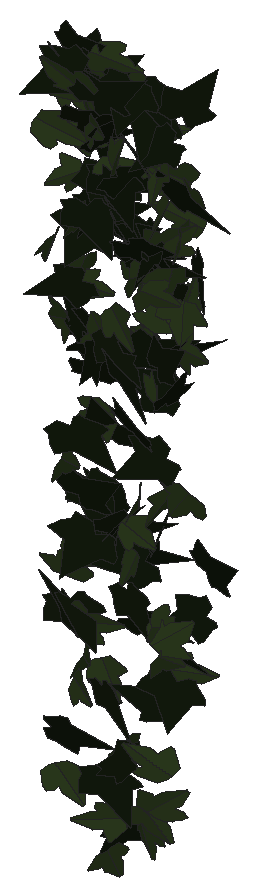
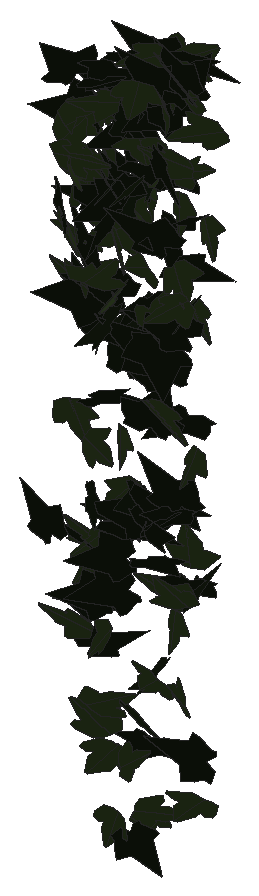
# SketchUp Ruby script. Lengths in inches.
U = 1.inch
M = Sketchup.active_model
def pt(a) = Geom::Point3d.new(a.map { |v| v * U })
def face(e, loops, mat)
  f = e.add_face(loops[0].map { |a| pt(a) })
  loops[1..].each { |l| e.add_face(l.map { |a| pt(a) }).erase! }
  f.material = f.back_material = mat if mat
  f
end
# faces: each face lists its corners as indices into pts; further lists are holes
def faces(e, pts, list, mat = nil) = list.each { |f| face(e, (f[0].is_a?(Array) ? f : [f]).map { |l| l.map { |i| pts[i] } }, mat) }
# xy, xz, yz: faces in a plane at the given z, y or x. An outline is a flat list of corners, or four numbers for a rectangle; further outlines are holes
def ring(l) = l.size == 4 ? [[l[0], l[1]], [l[2], l[1]], [l[2], l[3]], [l[0], l[3]]] : l.each_slice(2).to_a
def flat(e, list, mat, &to3) = list.each { |f| face(e, (f[0].is_a?(Array) ? f : [f]).map { |l| ring(l).map { |u, v| to3.(u, v) } }, mat) }
def xy(e, z, list, mat = nil) = flat(e, list, mat) { |x, y| [x, y, z] }
def xz(e, y, list, mat = nil) = flat(e, list, mat) { |x, z| [x, y, z] }
def yz(e, x, list, mat = nil) = flat(e, list, mat) { |y, z| [x, y, z] }
def lines(e, pts, list) = list.each { |a, b| e.add_line(pt(pts[a]), pt(pts[b])) }
# prism: a flat outline (further loops are holes) pulled along v
def prism(e, loops, v, mat = nil)
  f = face(e, loops, mat); d = Geom::Vector3d.new(v.map { |x| x * U })
  f.pushpull(f.normal.samedirection?(d) ? d.length : -d.length)
end
def box(e, o, s, mat = nil) = prism(e, [[o, [o[0] + s[0], o[1], o[2]], [o[0] + s[0], o[1] + s[1], o[2]], [o[0], o[1] + s[1], o[2]]]], [0, 0, s[2]], mat)
def at(x, y, z, deg = 0) = Geom::Transformation.translation(pt([x, y, z])) * Geom::Transformation.rotation(ORIGIN, Z_AXIS, deg.degrees)
def axes(o, x, y, z) = Geom::Transformation.new([*x, 0, *y, 0, *z, 0, *pt(o).to_a, 1])
def part(name) = M.definitions.add(name)
# library, detail: a bought-in or finely detailed component or shape, given as its bounding box
def library(name, o, s) = part(name).tap { |d| box(d.entities, o, s) }
def detail(e, o, s) = box(e.add_group.entities, o, s)
def put(e, d, t, mat = nil) = e.add_instance(d, t).tap { |i| i.material = mat if mat }
def group(e, t, mat = nil) = e.add_group.tap { |g| g.transformation = t; g.material = mat if mat }.entities
root = M.entities
M.materials.add("1026 AP 7946 SUNNY SIDE UP").color = [254, 231, 186]
M.materials.add("efeu1").color = [18, 25, 13]
M.materials.add("efeu2").color = [43, 57, 29]
c1 = part("ivyleaf_10")
p = [[0,0.5,-0.03],[-0.0625,2.02,-0.43],[-0.19,2.01,-0.46],[-0.54,1.05,-0.29],[-0.52,0.625,-0.18],[-0.83,0.76,-0.28],
  [-1.16,0.64,-0.33],[-1.15,0.33,-0.24],[-0.77,-0.39,0.02],[-0.3,-0.51,0.16],[0.04,-0.48,0.23],[-0.02,2.01,-0.4375],
  [-0.06,2.01,-0.43],[0.04,-0.49,0.23],[0.67,-0.49,0.14],[1.38,0.36,-0.2],[1.375,0.51,-0.24],[0.81,0.65,-0.19],
  [0.62,0.59,-0.15],[0.6,1.09,-0.28],[0.5,1.23,-0.31]]
faces(c1.entities,p,[[0,1,2,3,4,5,6,7,8,9,10],[11,12,0,13,14,15,16,17,18,19,20]],"efeu2")
c2 = part("ivyleaf_9")
p = [[1.54,2.16,1.25],[1.36,2.04,1.19],[-0.21,0.99,0.68],[-0.71,1.11,0.82],[-0.85,0.86,0.67],[-0.8,0.17,0.21],
  [-0.9,-0.01,0.1],[-0.67,-0.16,-0.02],[-0.08,-0.08,-0.05],[-0.03,-0.6,-0.4],[0.65,-0.88,-0.66],[0.83,-0.6,-0.49],
  [1.29,-0.42,-0.43],[1.8125,-0.07,-0.26],[1.21,0.44,0.15]]
faces(c2.entities,p,[[0,1,2,3,4,5,6,7,8,9,10,11,12,13,14]],"efeu1")
put(root,c1,axes([122.13,211.3,257.38],[0.35645,-0.04981,-0.17052],[0.27101,0.05135,0.22795],[-0.01392,-0.27578,0.07152]),"1026 AP 7946 SUNNY SIDE UP")
put(root,c2,axes([121.31,211.42,257.96],[0.17146,-0.27843,-0.07067],[-0.03874,0.06232,-0.30768],[0.44863,0.11179,0.00044]),"1026 AP 7946 SUNNY SIDE UP")
put(root,c1,axes([119.7,211.37,264.34],[0.01738,-0.26646,-0.03839],[-0.00826,0.03556,-0.27451],[0.42266,0.01165,-0.00378]),"1026 AP 7946 SUNNY SIDE UP")
put(root,c2,axes([120.48,211.53,258.76],[-0.41203,-0.1555,-0.01385],[0.03677,-0.01487,-0.31296],[0.24253,-0.26192,0.02391]),"1026 AP 7946 SUNNY SIDE UP")
put(root,c2,axes([121.37,211.48,261.125],[0.2981,-0.19969,0.09121],[-0.07262,0.07947,0.28337],[-0.33646,-0.19408,0.01965]),"1026 AP 7946 SUNNY SIDE UP")
put(root,c1,axes([120.26,211.42,267.41],[-0.31232,-0.00425,-0.24904],[-0.38005,0.01007,0.20449],[0.00798,0.3127,-0.00814]),"1026 AP 7946 SUNNY SIDE UP")
put(root,c2,axes([120.09,211.42,257.38],[-0.12685,-0.19199,-0.18978],[0.16044,0.15423,-0.21199],[0.38511,-0.1275,0.02581]),"1026 AP 7946 SUNNY SIDE UP")
put(root,c1,axes([121.87,211.27,264.08],[-0.14592,-0.12417,-0.227],[0.2458,0.1554,-0.15764],[0.31141,-0.18084,0.01806]),"1026 AP 7946 SUNNY SIDE UP")
put(root,c2,axes([120.45,211.4375,265.16],[-0.1716,-0.15631,-0.2075],[0.22646,0.14183,-0.19381],[0.32947,-0.1789,0.02514]),"1026 AP 7946 SUNNY SIDE UP")
put(root,c2,axes([122.17,211.42,262],[0.17485,0.22052,0.14723],[-0.12657,-0.11771,0.25318],[0.39221,-0.1363,0.01607]),"1026 AP 7946 SUNNY SIDE UP")
put(root,c1,axes([120.93,211.51,263.18],[0.24339,-0.03702,0.2455],[0.35729,-0.07323,-0.16405],[0.12803,0.27475,-0.0089]),"1026 AP 7946 SUNNY SIDE UP")
put(root,c2,axes([120.03,211.48,257.06],[0.04907,-0.27723,0.11257],[-0.00652,0.11104,0.28794],[-0.46942,-0.03052,0.00776]),"1026 AP 7946 SUNNY SIDE UP")
put(root,c2,axes([121,211.56,262.22],[0.20229,-0.2839,0.08219],[0.03043,-0.08048,-0.3212],[0.4634,0.12922,-0.01479]),"1026 AP 7946 SUNNY SIDE UP")
put(root,c1,axes([122.17,211.29,257.08],[-0.08076,-0.16814,-0.23165],[0.13908,0.20625,-0.17925],[0.41775,-0.10117,0.01489]),"1026 AP 7946 SUNNY SIDE UP")
put(root,c1,axes([120.43,211.31,256.48],[-0.00739,-0.21195,-0.2007],[0.0039,0.19361,-0.21727],[0.45138,-0.00514,-0.00141]),"1026 AP 7946 SUNNY SIDE UP")
put(root,c2,axes([120.11,211.61,263.54],[-0.05413,-0.04797,-0.26856],[-0.07871,-0.25669,0.05403],[-0.40886,0.05577,0.02515]),"1026 AP 7946 SUNNY SIDE UP")
put(root,c2,axes([120.37,211.68,262.18],[0.05543,-0.10242,-0.26572],[0.29351,-0.18288,0.10025],[-0.32177,-0.18446,0.04567]),"1026 AP 7946 SUNNY SIDE UP")
put(root,c2,axes([121.89,211.54,262.52],[-0.07735,0.11038,0.25409],[0.1593,-0.22419,0.12318],[0.39292,0.11262,0.00008]),"1026 AP 7946 SUNNY SIDE UP")
put(root,c1,axes([121.98,211.54,265.63],[0.19412,-0.29203,0.00351],[-0.0127,-0.00891,-0.32648],[0.45907,0.12323,-0.01051]),"1026 AP 7946 SUNNY SIDE UP")
put(root,c1,axes([119.97,211.5,257.91],[-0.42821,-0.04133,0.03396],[0.04542,0.02998,0.28275],[-0.06989,0.2727,-0.02429]),"1026 AP 7946 SUNNY SIDE UP")
put(root,c1,axes([120.25,211.45,257.01],[-0.1746,-0.02185,0.27982],[0.39764,0.10136,0.11544],[-0.16014,0.2755,-0.01844]),"1026 AP 7946 SUNNY SIDE UP")
put(root,c2,axes([121.75,211.62,264.78],[-0.29529,0.04858,-0.19804],[0.26416,-0.10235,-0.19604],[-0.1664,-0.2487,0.04023]),"1026 AP 7946 SUNNY SIDE UP")
put(root,c2,axes([122.2,211.63,256.43],[-0.314,-0.1852,-0.09814],[0.12893,0.04983,-0.27966],[0.30021,-0.21511,0.01746]),"1026 AP 7946 SUNNY SIDE UP")
put(root,c1,axes([120.25,211.66,266.65],[-0.09219,0.06354,0.3122],[0.40424,-0.16127,0.08523],[0.27038,0.26278,-0.02098]),"1026 AP 7946 SUNNY SIDE UP")
put(root,c1,axes([121.9,211.46,253.96],[-0.2758,-0.14185,0.18032],[0.19242,0.12749,0.23244],[-0.29863,0.21315,-0.01677]),"1026 AP 7946 SUNNY SIDE UP")
put(root,c2,axes([120.58,211.46,267.29],[-0.09726,0.0188,0.29021],[0.43638,-0.04833,0.06584],[0.08064,0.28423,-0.00629]),"1026 AP 7946 SUNNY SIDE UP")
put(root,c2,axes([120.09,211.68,267.6],[-0.45384,-0.07922,0.10622],[-0.14375,-0.05639,-0.30727],[0.14618,-0.30142,0.02762]),"1026 AP 7946 SUNNY SIDE UP")
put(root,c2,axes([121.41,211.41,264.76],[0.4568,0.10388,0.03026],[0.05796,-0.01798,-0.31652],[-0.15928,0.29138,-0.0284]),"1026 AP 7946 SUNNY SIDE UP")
put(root,c2,axes([120.76,211.57,254.16],[-0.17763,-0.16469,-0.20567],[0.21144,0.14758,-0.2039],[0.34638,-0.17454,0.01899]),"1026 AP 7946 SUNNY SIDE UP")
put(root,c1,axes([120.86,211.49,252.6875],[-0.15712,-0.23477,-0.1245],[0.09723,0.10335,-0.2618],[0.40266,-0.11657,0.01464]),"1026 AP 7946 SUNNY SIDE UP")
put(root,c1,axes([122.07,211.61,264.36],[-0.22024,-0.26846,0.02961],[-0.00042,-0.03395,-0.31174],[0.42481,-0.13922,0.01504]),"1026 AP 7946 SUNNY SIDE UP")
put(root,c1,axes([121.98,211.38,257.58],[-0.00373,-0.10392,-0.2924],[0.19225,0.25862,-0.0973],[0.4337,-0.11553,0.04061]),"1026 AP 7946 SUNNY SIDE UP")
put(root,c1,axes([119.87,211.79,265.5],[-0.07928,-0.01146,0.2649],[-0.03681,-0.26079,-0.01822],[0.40314,-0.02606,0.05043]),"1026 AP 7946 SUNNY SIDE UP")
put(root,c2,axes([121.21,211.59,254.6],[-0.34744,0.17726,0.01238],[-0.03685,-0.01168,-0.29087],[-0.27682,-0.22093,0.02319]),"1026 AP 7946 SUNNY SIDE UP")
put(root,c1,axes([121,211.4,266.28],[-0.01135,0.04937,-0.29232],[-0.00066,0.28412,0.05255],[0.45331,0.00165,-0.00724]),"1026 AP 7946 SUNNY SIDE UP")
put(root,c2,axes([120,211.5625,260.66],[-0.04346,-0.13668,-0.2638],[0.17624,0.23142,-0.13878],[0.41985,-0.11129,0.03095]),"1026 AP 7946 SUNNY SIDE UP")
put(root,c1,axes([121.17,211.7,258.46],[0.28319,-0.1996,0.03504],[0.01638,-0.03784,-0.27659],[0.31825,0.17955,-0.01694]),"1026 AP 7946 SUNNY SIDE UP")
put(root,c1,axes([121.44,211.51,259.79],[0.02966,-0.21179,-0.19625],[-0.03492,0.18803,-0.21791],[0.44528,0.02885,-0.00402]),"1026 AP 7946 SUNNY SIDE UP")
put(root,c1,axes([119.8125,211.53,262.75],[0.18328,-0.09495,-0.24688],[-0.19858,0.20758,-0.14713],[0.35244,0.16634,0.04549]),"1026 AP 7946 SUNNY SIDE UP")
put(root,c2,axes([120.79,211.65,262.67],[0.08645,-0.24476,-0.16612],[-0.04859,0.15689,-0.25749],[0.45711,0.06297,0.00405]),"1026 AP 7946 SUNNY SIDE UP")
put(root,c2,axes([121.74,211.86,260.54],[-0.30614,-0.13274,0.16842],[-0.17564,-0.12484,-0.24109],[0.28179,-0.22202,0.03269]),"1026 AP 7946 SUNNY SIDE UP")
put(root,c2,axes([120.76,211.72,265.78],[-0.24118,-0.08477,-0.25373],[0.35962,0.09178,-0.17909],[0.19449,-0.27482,0.01651]),"1026 AP 7946 SUNNY SIDE UP")
put(root,c2,axes([121.02,211.71,264.64],[-0.05196,0.07812,0.26513],[0.2502,-0.20282,0.08343],[0.34012,0.16113,-0.02087]),"1026 AP 7946 SUNNY SIDE UP")
put(root,c1,axes([121.57,211.63,253.6875],[-0.36864,-0.08016,-0.13786],[0.2148,0.00944,-0.25318],[0.11715,-0.26955,0.03041]),"1026 AP 7946 SUNNY SIDE UP")
put(root,c1,axes([121.66,211.79,266.22],[0.35977,-0.14787,0.12418],[0.12803,-0.09597,-0.27912],[0.27221,0.24057,-0.03285]),"1026 AP 7946 SUNNY SIDE UP")
put(root,c1,axes([121.79,211.74,254.56],[0.19521,0.13661,0.22047],[-0.27055,-0.12875,0.18742],[0.29218,-0.21049,0.02624]),"1026 AP 7946 SUNNY SIDE UP")
put(root,c1,axes([121.37,211.49,264.13],[-0.02439,-0.09403,-0.28159],[0.10394,0.26478,-0.09634],[0.44166,-0.06751,0.00712]),"1026 AP 7946 SUNNY SIDE UP")
put(root,c2,axes([120.02,211.92,264.47],[-0.19396,-0.24852,0.10778],[-0.0472,-0.10324,-0.28584],[0.42222,-0.12571,0.01756]),"1026 AP 7946 SUNNY SIDE UP")
put(root,c1,axes([120.08,211.62,264.8],[0.00528,-0.24485,-0.15836],[-0.01151,0.15221,-0.25133],[0.45328,0.00672,-0.00454]),"1026 AP 7946 SUNNY SIDE UP")
put(root,c2,axes([120.04,211.71,266.5625],[0.44392,0.1069,-0.05883],[0.06361,0.05494,0.30905],[0.18012,-0.28287,0.03584]),"1026 AP 7946 SUNNY SIDE UP")
put(root,c1,axes([119.42,211.59,266.36],[0.14175,0.09213,0.27759],[0.30948,0.18334,-0.1316],[-0.32253,0.21642,-0.00427]),"1026 AP 7946 SUNNY SIDE UP")
put(root,c2,axes([121.28,211.67,264.35],[0.25729,-0.00119,0.26048],[0.39004,-0.05765,-0.16599],[0.0771,0.29561,-0.02953]),"1026 AP 7946 SUNNY SIDE UP")
put(root,c2,axes([121.92,211.77,265.91],[0.37389,-0.11974,0.19695],[0.23469,-0.12607,-0.27236],[0.26717,0.27831,-0.03637]),"1026 AP 7946 SUNNY SIDE UP")
put(root,c1,axes([122.36,211.71,260.0625],[-0.39065,0.01733,0.14657],[-0.22512,-0.02185,-0.25512],[-0.00648,-0.28541,0.02674]),"1026 AP 7946 SUNNY SIDE UP")
put(root,c2,axes([121.78,211.85,255.73],[-0.07358,0.01305,0.27558],[-0.40172,-0.0834,-0.04235],[0.12596,-0.25836,0.02591]),"1026 AP 7946 SUNNY SIDE UP")
put(root,c2,axes([120.47,211.8125,255.63],[0.19614,-0.25391,-0.00511],[-0.01623,-0.00115,-0.29127],[0.39895,0.12478,-0.00934]),"1026 AP 7946 SUNNY SIDE UP")
put(root,c1,axes([119.78,211.59,259.96],[-0.03187,-0.1885,-0.22565],[0.07858,0.21289,-0.19321],[0.44625,-0.05095,0.01791]),"1026 AP 7946 SUNNY SIDE UP")
put(root,c2,axes([122.65,211.8,257.8],[-0.43565,0.07384,0.04147],[-0.07168,-0.01711,-0.29408],[-0.11075,-0.27939,0.02722]),"1026 AP 7946 SUNNY SIDE UP")
put(root,c1,axes([121.87,211.68,264.82],[-0.25959,-0.18712,0.18065],[0.1916,0.1277,0.25776],[-0.35611,0.20511,0.00699]),"1026 AP 7946 SUNNY SIDE UP")
put(root,c2,axes([120.99,211.93,267.48],[-0.24713,-0.24664,-0.00411],[0.0267,-0.00775,-0.30073],[0.38692,-0.15699,0.01812]),"1026 AP 7946 SUNNY SIDE UP")
put(root,c2,axes([121.39,211.64,262.54],[0.0328,0.03535,0.29277],[0.44129,0.05322,-0.02775],[-0.0881,0.27974,-0.02999]),"1026 AP 7946 SUNNY SIDE UP")
put(root,c2,axes([119.81,211.8,267.16],[0.22088,-0.16043,0.18184],[-0.1561,0.1481,0.21979],[-0.34219,-0.17111,0.01711]),"1026 AP 7946 SUNNY SIDE UP")
put(root,c2,axes([120.02,211.75,262.54],[-0.06244,-0.21679,0.17166],[0.04073,0.16589,0.22799],[-0.42919,0.04728,-0.00334]),"1026 AP 7946 SUNNY SIDE UP")
put(root,c1,axes([120.42,211.89,262.46],[-0.2118,-0.21418,-0.12595],[-0.12551,-0.09249,0.25956],[-0.36592,0.15569,-0.01612]),"1026 AP 7946 SUNNY SIDE UP")
put(root,c1,axes([120.11,211.79,267.43],[-0.30993,-0.19682,-0.00897],[0.02903,-0.00776,-0.28637],[0.30835,-0.1971,0.01794]),"1026 AP 7946 SUNNY SIDE UP")
put(root,c2,axes([121.01,211.58,265.88],[0.00619,0.05657,-0.29499],[0.04001,0.28553,0.06008],[0.4577,-0.02572,-0.00126]),"1026 AP 7946 SUNNY SIDE UP")
put(root,c2,axes([121.22,211.92,258.34],[-0.08501,-0.08981,-0.27451],[-0.25584,-0.21067,0.10613],[-0.35967,0.17108,-0.01062]),"1026 AP 7946 SUNNY SIDE UP")
put(root,c1,axes([122.13,211.85,263.59],[0.44215,-0.02151,0.06214],[0.09095,-0.03255,-0.28934],[0.04364,0.28577,-0.02658]),"1026 AP 7946 SUNNY SIDE UP")
put(root,c2,axes([121.9,211.83,261.9],[-0.2865,-0.11011,-0.20164],[-0.27535,-0.08686,0.21846],[-0.21972,0.25243,-0.01085]),"1026 AP 7946 SUNNY SIDE UP")
put(root,c1,axes([119.64,211.87,267.1],[0.2029,0.01063,0.2757],[0.41882,-0.03557,-0.13109],[0.04321,0.29491,-0.024]),"1026 AP 7946 SUNNY SIDE UP")
put(root,c2,axes([120.45,211.58,266.45],[0.17204,0.18087,0.22449],[0.21808,0.1682,-0.2156],[-0.38682,0.17527,-0.0217]),"1026 AP 7946 SUNNY SIDE UP")
put(root,c2,axes([121.53,211.92,264.57],[0.00114,-0.29796,0.06402],[0.02992,0.06375,0.30672],[-0.47821,0.00328,0.01934]),"1026 AP 7946 SUNNY SIDE UP")
put(root,c2,axes([121.86,211.9,266.71],[-0.42183,0.04041,-0.03425],[0.0458,-0.03042,-0.27842],[-0.06865,-0.26863,0.02475]),"1026 AP 7946 SUNNY SIDE UP")
put(root,c1,axes([121.71,211.99,259.73],[0.01108,-0.232,0.17012],[0.00171,-0.16648,-0.24007],[0.44897,0.00636,-0.00329]),"1026 AP 7946 SUNNY SIDE UP")
put(root,c2,axes([120.72,211.96,264.67],[0.20778,-0.23724,0.08311],[0.05073,-0.07587,-0.28007],[0.39143,0.13577,-0.00781]),"1026 AP 7946 SUNNY SIDE UP")
put(root,c1,axes([119.73,211.98,255.41],[0.04704,0.0149,0.26967],[0.36084,-0.12873,-0.02023],[0.19911,0.22978,-0.02705]),"1026 AP 7946 SUNNY SIDE UP")
put(root,c2,axes([120.875,212.05,266.23],[0.06852,-0.17312,0.22521],[0.12377,-0.20566,-0.18433],[0.4219,0.08845,0.0175]),"1026 AP 7946 SUNNY SIDE UP")
put(root,c1,axes([120.55,212,253.05],[0.08153,0.00181,-0.27145],[-0.35412,-0.13913,-0.04745],[-0.21512,0.22971,-0.02477]),"1026 AP 7946 SUNNY SIDE UP")
put(root,c2,axes([119.88,211.92,259.17],[-0.09396,-0.00447,0.29762],[0.35642,-0.18371,0.0443],[0.28179,0.23087,0.04321]),"1026 AP 7946 SUNNY SIDE UP")
put(root,c1,axes([120.69,211.92,265.86],[0.32264,0.16743,-0.04643],[-0.03594,-0.04458,-0.27233],[-0.27066,0.20551,-0.01919]),"1026 AP 7946 SUNNY SIDE UP")
put(root,c1,axes([121.1,211.74,259.02],[0.07378,0.19775,0.18627],[0.06844,0.17434,-0.20835],[-0.41453,0.06398,-0.00125]),"1026 AP 7946 SUNNY SIDE UP")
put(root,c1,axes([121.99,212,262.74],[0.03713,-0.0432,-0.293],[0.34318,-0.18284,0.04625],[-0.2941,-0.21881,0.01698]),"1026 AP 7946 SUNNY SIDE UP")
put(root,c2,axes([120.46,212.02,265.52],[-0.3182,-0.22029,-0.07706],[0.103,0.03945,-0.30718],[0.35036,-0.21167,0.02032]),"1026 AP 7946 SUNNY SIDE UP")
put(root,c1,axes([122.04,212.07,264.99],[0.13034,-0.16043,0.23049],[0.14843,-0.20394,-0.18711],[0.40789,0.12548,-0.00556]),"1026 AP 7946 SUNNY SIDE UP")
put(root,c2,axes([120.4375,211.97,260.52],[0.34778,-0.04863,0.17284],[-0.24591,0.06647,0.23224],[-0.12331,-0.26971,0.02434]),"1026 AP 7946 SUNNY SIDE UP")
put(root,c2,axes([121.15,211.72,264.47],[0.27992,0.14998,0.18037],[0.2413,0.08656,-0.23778],[-0.26916,0.23357,-0.02559]),"1026 AP 7946 SUNNY SIDE UP")
put(root,c1,axes([121.65,211.73,261.8],[0.01438,0.17078,-0.23494],[-0.05009,0.22833,0.17543],[0.44642,0.02012,0.02725]),"1026 AP 7946 SUNNY SIDE UP")
put(root,c2,axes([120.68,211.93,265.19],[0.23906,-0.22872,-0.10672],[-0.09359,0.08326,-0.28243],[0.3827,0.16324,-0.0024]),"1026 AP 7946 SUNNY SIDE UP")
put(root,c1,axes([120.63,211.74,264.81],[-0.04497,0.09244,-0.27805],[-0.14922,0.25328,0.10101],[0.42388,0.09897,0.00606]),"1026 AP 7946 SUNNY SIDE UP")
put(root,c2,axes([119.78,211.89,262.4375],[0.16903,-0.02634,0.26354],[0.39437,-0.05131,-0.11425],[0.09047,0.27285,0.00563]),"1026 AP 7946 SUNNY SIDE UP")
put(root,c1,axes([119.86,212,263.68],[-0.11191,-0.29232,0.03332],[-0.00019,-0.03495,-0.31004],[0.46275,-0.07071,0.00793]),"1026 AP 7946 SUNNY SIDE UP")
put(root,c2,axes([119.33,211.9375,254.41],[0.24218,0.05166,-0.23121],[0.30783,0.1135,0.16576],[0.19158,-0.24767,0.02592]),"1026 AP 7946 SUNNY SIDE UP")
put(root,c1,axes([120.33,211.96,260.87],[0.32108,-0.12091,-0.1886],[-0.2681,0.06844,-0.243],[0.21566,0.2651,-0.0213]),"1026 AP 7946 SUNNY SIDE UP")
put(root,c2,axes([120.75,211.75,258.85],[-0.11341,0.18139,-0.1911],[-0.12157,0.16988,0.20198],[0.39063,0.10553,0.00738]),"1026 AP 7946 SUNNY SIDE UP")
put(root,c1,axes([121.97,212.125,265.94],[-0.16044,-0.08866,-0.26071],[-0.30804,-0.15945,0.13826],[-0.28681,0.22085,-0.00266]),"1026 AP 7946 SUNNY SIDE UP")
put(root,c1,axes([121.3125,212.08,262.53],[-0.17124,0.20861,0.14632],[-0.00249,-0.15404,0.23286],[0.39579,0.08929,0.06478]),"1026 AP 7946 SUNNY SIDE UP")
put(root,c2,axes([120.09,211.77,267.1875],[0.20938,0.19157,0.15783],[0.15567,0.11617,-0.23932],[-0.35174,0.16545,-0.01197]),"1026 AP 7946 SUNNY SIDE UP")
put(root,c2,axes([120.06,212.02,261.5625],[0.40892,0.08884,0.03987],[-0.06962,0.01195,0.28197],[0.13518,-0.26258,0.0246]),"1026 AP 7946 SUNNY SIDE UP")
put(root,c1,axes([121.14,211.97,264.06],[-0.32409,-0.05007,-0.1937],[0.29781,0.0093,-0.21671],[0.06819,-0.27864,0.02589]),"1026 AP 7946 SUNNY SIDE UP")
put(root,c2,axes([121.47,212.01,256.83],[0.34153,-0.06936,0.15035],[0.2036,-0.07265,-0.23389],[0.15293,0.25162,-0.02438]),"1026 AP 7946 SUNNY SIDE UP")
put(root,c1,axes([119.42,211.96,253.58],[0.29865,0.1449,0.14662],[0.18867,0.07578,-0.24541],[-0.25655,0.2244,-0.00979]),"1026 AP 7946 SUNNY SIDE UP")
put(root,c1,axes([120.48,212.1875,264.65],[0.15302,-0.2008,0.17459],[0.09234,-0.16077,-0.23038],[0.4039,0.11283,-0.01348]),"1026 AP 7946 SUNNY SIDE UP")
put(root,c2,axes([121.3,212.18,266.95],[-0.27854,-0.22115,-0.02878],[0.05113,0.00805,-0.29111],[0.34651,-0.17896,0.01983]),"1026 AP 7946 SUNNY SIDE UP")
put(root,c2,axes([121.03,211.9375,257.125],[0.35462,0.06313,0.15507],[0.23896,0.01082,-0.23974],[-0.09224,0.27073,-0.02491]),"1026 AP 7946 SUNNY SIDE UP")
put(root,c2,axes([120.27,211.98,261.9],[0.31195,0.20425,-0.1091],[0.09318,0.09133,0.29316],[0.35044,-0.2061,0.01916]),"1026 AP 7946 SUNNY SIDE UP")
put(root,c2,axes([121.56,212.21,263.47],[-0.04148,0.08156,0.30969],[0.1096,-0.29202,0.08635],[0.47664,0.07425,0.00709]),"1026 AP 7946 SUNNY SIDE UP")
put(root,c1,axes([122.13,212.05,263.64],[0.32402,-0.20016,0.03429],[-0.01623,0.03865,0.29543],[-0.31895,-0.20532,0.0198]),"1026 AP 7946 SUNNY SIDE UP")
put(root,c2,axes([120.54,211.91,258.67],[0.16298,0.0398,0.29717],[0.4252,0.09978,-0.11379],[-0.1689,0.2896,0.00029]),"1026 AP 7946 SUNNY SIDE UP")
put(root,c2,axes([122.13,212.27,264.33],[-0.05767,-0.03161,-0.32053],[0.46039,-0.11306,-0.0244],[-0.17202,-0.29199,0.04216]),"1026 AP 7946 SUNNY SIDE UP")
put(root,c1,axes([122.17,212.13,265.17],[0.09139,0.06566,0.28604],[-0.42007,-0.08589,0.07814],[0.15588,-0.26997,0.04288]),"1026 AP 7946 SUNNY SIDE UP")
put(root,c1,axes([121.15,212.03,263.93],[0.15148,-0.20882,-0.17105],[-0.10087,0.15192,-0.23599],[0.40599,0.11566,0.00519]),"1026 AP 7946 SUNNY SIDE UP")
put(root,c1,axes([121.47,211.92,256.11],[-0.00867,0.07765,0.27695],[-0.13271,0.25544,-0.07642],[-0.4188,-0.08255,0.01849]),"1026 AP 7946 SUNNY SIDE UP")
put(root,c2,axes([120.18,212.06,262.16],[0.21526,0.24067,-0.11229],[-0.06922,-0.10182,-0.28561],[-0.41053,0.14336,-0.01072]),"1026 AP 7946 SUNNY SIDE UP")
put(root,c1,axes([120.15,212.21,255.78],[0.3256,0.00452,0.17374],[0.26301,-0.04003,-0.21074],[0.0343,0.26403,-0.03334]),"1026 AP 7946 SUNNY SIDE UP")
put(root,c2,axes([119.97,211.91,264.2],[0.071,0.06521,0.29624],[0.23249,0.24625,-0.08011],[-0.40047,0.15452,0.00601]),"1026 AP 7946 SUNNY SIDE UP")
put(root,c2,axes([119.46,212.25,267.52],[-0.03975,0.02707,0.28732],[0.24139,-0.23275,0.03627],[0.36832,0.15546,0.00724]),"1026 AP 7946 SUNNY SIDE UP")
put(root,c2,axes([121.79,211.93,262.52],[0.02089,0.23196,-0.21166],[0.00206,0.20692,0.24043],[0.48861,-0.01079,0.00803]),"1026 AP 7946 SUNNY SIDE UP")
put(root,c1,axes([121.58,212.16,263.01],[0.33554,0.19119,0.12931],[-0.18127,-0.05666,0.293],[0.30952,-0.24044,0.03141]),"1026 AP 7946 SUNNY SIDE UP")
put(root,c1,axes([120.2,212.08,267.78],[-0.16103,-0.09022,-0.25716],[0.36018,0.10406,-0.13523],[0.20935,-0.24843,0.03485]),"1026 AP 7946 SUNNY SIDE UP")
put(root,c1,axes([122.125,212.15,265.57],[-0.36547,0.09087,-0.14554],[-0.19346,0.07339,0.25666],[0.18082,0.26218,-0.01957]),"1026 AP 7946 SUNNY SIDE UP")
put(root,c2,axes([119.82,212.3,259.0625],[-0.04463,-0.26064,-0.02783],[0.00949,0.02502,-0.26993],[0.41168,-0.02884,0.00321]),"1026 AP 7946 SUNNY SIDE UP")
put(root,c2,axes([120.04,212.16,267.26],[-0.11538,0.00761,0.2799],[0.41807,-0.05623,0.07528],[0.08845,0.27572,0.00931]),"1026 AP 7946 SUNNY SIDE UP")
put(root,c1,axes([119.82,212.375,266.9375],[-0.11924,0.06,-0.26585],[0.12939,-0.25018,-0.08619],[-0.39655,-0.09967,0.05182]),"1026 AP 7946 SUNNY SIDE UP")
put(root,c2,axes([120.96,212.24,267.32],[-0.14705,-0.18693,-0.23245],[0.24755,0.16641,-0.20926],[0.38706,-0.17745,0.04552]),"1026 AP 7946 SUNNY SIDE UP")
put(root,c1,axes([121.76,212.22,256.28],[0.10283,-0.06265,-0.26515],[0.40863,-0.03431,0.07654],[-0.07781,-0.26298,0.05153]),"1026 AP 7946 SUNNY SIDE UP")
put(root,c1,axes([119.71,212.1,263.14],[-0.12088,-0.11564,-0.25136],[0.27065,0.17359,-0.13999],[0.3259,-0.18705,0.02302]),"1026 AP 7946 SUNNY SIDE UP")
put(root,c2,axes([121.16,212.17,264.34],[0.12515,-0.1496,-0.22388],[-0.18844,0.18073,-0.17301],[0.36835,0.14329,-0.01244]),"1026 AP 7946 SUNNY SIDE UP")
put(root,c2,axes([120.57,212.32,252.73],[-0.03861,0.18195,-0.20452],[0.04542,-0.19746,-0.19029],[-0.42219,-0.03788,-0.00177]),"1026 AP 7946 SUNNY SIDE UP")
put(root,c1,axes([119.55,212.28,265.98],[0.04372,-0.06792,-0.27625],[0.42876,-0.03638,0.03846],[-0.06961,-0.26674,0.0634]),"1026 AP 7946 SUNNY SIDE UP")
put(root,c2,axes([119.9,212.15,267.62],[-0.12505,0.18253,0.17922],[-0.13621,0.15038,-0.20368],[-0.37116,-0.11668,0.01437]),"1026 AP 7946 SUNNY SIDE UP")
put(root,c1,axes([121.1875,212.15,266.56],[0.07578,-0.01344,-0.28787],[0.33035,0.18886,0.02908],[0.29029,-0.21141,0.04205]),"1026 AP 7946 SUNNY SIDE UP")
put(root,c2,axes([119.73,212.32,259.23],[-0.0183,-0.19507,-0.18294],[0.0741,0.17224,-0.19833],[0.40692,-0.04014,0.02789]),"1026 AP 7946 SUNNY SIDE UP")
put(root,c1,axes([120.97,212.32,252.89],[-0.37295,0.13332,-0.01863],[0.00796,-0.0293,-0.27947],[-0.21157,-0.23612,0.02232]),"1026 AP 7946 SUNNY SIDE UP")
put(root,c2,axes([120.05,212.51,258.28],[-0.31637,-0.17471,0.0349],[-0.01982,-0.03851,-0.27392],[0.27944,-0.20054,0.02009]),"1026 AP 7946 SUNNY SIDE UP")
put(root,c2,axes([121,212.41,262.45],[0.29127,-0.25653,-0.02868],[-0.04757,0.01064,-0.32537],[0.4027,0.18681,-0.01769]),"1026 AP 7946 SUNNY SIDE UP")
put(root,c1,axes([120.52,212.57,254.22],[-0.02606,0.01387,-0.27761],[-0.13592,-0.2561,-0.0096],[-0.40205,0.08568,0.02124]),"1026 AP 7946 SUNNY SIDE UP")
put(root,c2,axes([121.32,212.53,259.06],[-0.1832,0.07329,-0.24334],[0.28157,-0.15576,-0.14145],[-0.26913,-0.21285,0.01765]),"1026 AP 7946 SUNNY SIDE UP")
put(root,c2,axes([122.12,212.59,258.16],[-0.03682,-0.00183,0.30881],[0.22938,-0.26275,0.00855],[0.41179,0.14619,0.02285]),"1026 AP 7946 SUNNY SIDE UP")
put(root,c2,axes([120.02,212.39,266.04],[0.04024,-0.03422,-0.28532],[-0.4361,0.02595,-0.02957],[0.04587,0.27673,-0.03086]),"1026 AP 7946 SUNNY SIDE UP")
put(root,c2,axes([119.82,212.45,264.43],[0.01044,0.02406,0.29028],[0.42384,-0.08534,0.00047],[0.1338,0.26848,-0.02412]),"1026 AP 7946 SUNNY SIDE UP")
put(root,c1,axes([119.43,212.43,257.66],[0.33042,0.03558,-0.16118],[0.23374,0.05474,0.21854],[0.09578,-0.25632,0.0227]),"1026 AP 7946 SUNNY SIDE UP")
put(root,c1,axes([120.33,212.49,267.26],[-0.34017,-0.14274,-0.04542],[0.07553,0.00551,-0.26606],[0.22204,-0.22056,0.02092]),"1026 AP 7946 SUNNY SIDE UP")
put(root,c2,axes([121.78,212.36,267.05],[-0.17238,-0.04935,0.29769],[0.39188,0.14732,0.12407],[-0.24354,0.27199,-0.01108]),"1026 AP 7946 SUNNY SIDE UP")
put(root,c2,axes([120.23,212.4,258.78],[-0.02589,0.04695,0.2711],[-0.21785,0.22366,-0.04878],[-0.35897,-0.13912,0.01005]),"1026 AP 7946 SUNNY SIDE UP")
put(root,c2,axes([120.6875,212.4,258.04],[0.23539,0.08032,0.21588],[0.3034,0.08149,-0.17408],[-0.17889,0.24391,-0.01119]),"1026 AP 7946 SUNNY SIDE UP")
